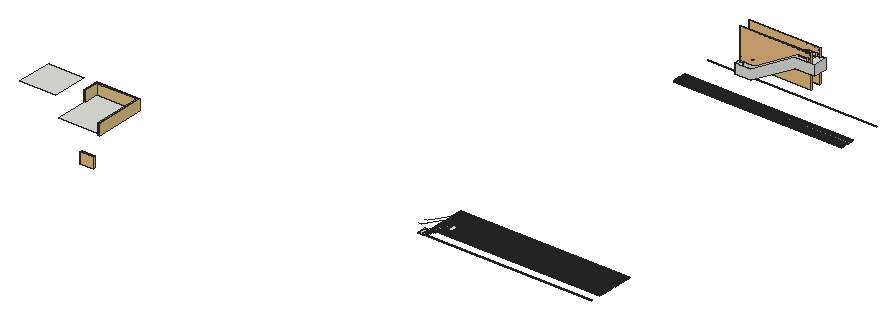
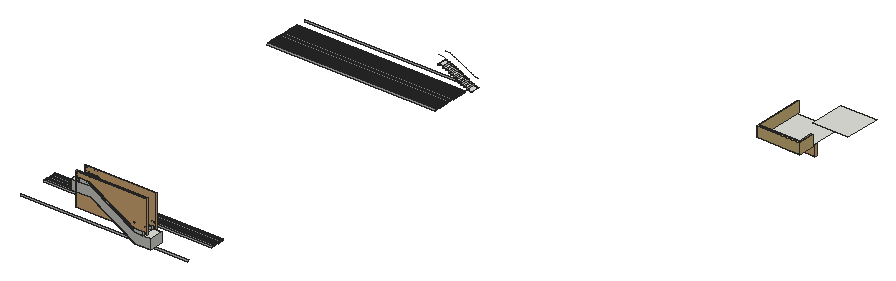
# SketchUp Ruby script. Lengths in inches.
U = 1.inch
M = Sketchup.active_model
def pt(a) = Geom::Point3d.new(a.map { |v| v * U })
def face(e, loops, mat)
  f = e.add_face(loops[0].map { |a| pt(a) })
  loops[1..].each { |l| e.add_face(l.map { |a| pt(a) }).erase! }
  f.material = f.back_material = mat if mat
  f
end
# faces: each face lists its corners as indices into pts; further lists are holes
def faces(e, pts, list, mat = nil) = list.each { |f| face(e, (f[0].is_a?(Array) ? f : [f]).map { |l| l.map { |i| pts[i] } }, mat) }
# xy, xz, yz: faces in a plane at the given z, y or x. An outline is a flat list of corners, or four numbers for a rectangle; further outlines are holes
def ring(l) = l.size == 4 ? [[l[0], l[1]], [l[2], l[1]], [l[2], l[3]], [l[0], l[3]]] : l.each_slice(2).to_a
def flat(e, list, mat, &to3) = list.each { |f| face(e, (f[0].is_a?(Array) ? f : [f]).map { |l| ring(l).map { |u, v| to3.(u, v) } }, mat) }
def xy(e, z, list, mat = nil) = flat(e, list, mat) { |x, y| [x, y, z] }
def xz(e, y, list, mat = nil) = flat(e, list, mat) { |x, z| [x, y, z] }
def yz(e, x, list, mat = nil) = flat(e, list, mat) { |y, z| [x, y, z] }
def lines(e, pts, list) = list.each { |a, b| e.add_line(pt(pts[a]), pt(pts[b])) }
# prism: a flat outline (further loops are holes) pulled along v
def prism(e, loops, v, mat = nil)
  f = face(e, loops, mat); d = Geom::Vector3d.new(v.map { |x| x * U })
  f.pushpull(f.normal.samedirection?(d) ? d.length : -d.length)
end
def box(e, o, s, mat = nil) = prism(e, [[o, [o[0] + s[0], o[1], o[2]], [o[0] + s[0], o[1] + s[1], o[2]], [o[0], o[1] + s[1], o[2]]]], [0, 0, s[2]], mat)
def at(x, y, z, deg = 0) = Geom::Transformation.translation(pt([x, y, z])) * Geom::Transformation.rotation(ORIGIN, Z_AXIS, deg.degrees)
def axes(o, x, y, z) = Geom::Transformation.new([*x, 0, *y, 0, *z, 0, *pt(o).to_a, 1])
def part(name) = M.definitions.add(name)
# library, detail: a bought-in or finely detailed component or shape, given as its bounding box
def library(name, o, s) = part(name).tap { |d| box(d.entities, o, s) }
def detail(e, o, s) = box(e.add_group.entities, o, s)
def put(e, d, t, mat = nil) = e.add_instance(d, t).tap { |i| i.material = mat if mat }
def group(e, t, mat = nil) = e.add_group.tap { |g| g.transformation = t; g.material = mat if mat }.entities
root = M.entities
M.materials.add("[Stone Brushed Khaki]").color = [226, 197, 133]
c1 = part("Group74\#1")
p = [[385.16,-763.86,0],[-385.16,-763.86,0],[-385.16,-767.25,5.875],[385.16,-767.25,5.875]]
faces(c1.entities,p,[[0,1,2,3]])
c2 = part("Group75\#1")
p = [[385.16,-759.92,0],[-385.16,-759.92,0],[-385.16,-763.3125,5.875],[385.16,-763.3125,5.875]]
faces(c2.entities,p,[[0,1,2,3]])
c3 = part("Group76\#1")
p = [[385.16,-755.98,0],[-385.16,-755.98,0],[-385.16,-759.375,5.875],[385.16,-759.375,5.875]]
faces(c3.entities,p,[[0,1,2,3]])
c4 = part("Group77\#1")
p = [[385.16,-752.05,0],[-385.16,-752.05,0],[-385.16,-755.4375,5.875],[385.16,-755.4375,5.875]]
faces(c4.entities,p,[[0,1,2,3]])
c5 = part("Group78\#1")
p = [[385.16,-748.11,0],[-385.16,-748.11,0],[-385.16,-751.5,5.875],[385.16,-751.5,5.875]]
faces(c5.entities,p,[[0,1,2,3]])
c6 = part("Group79\#1")
p = [[385.16,-744.17,0],[-385.16,-744.17,0],[-385.16,-747.5625,5.875],[385.16,-747.5625,5.875]]
faces(c6.entities,p,[[0,1,2,3]])
c7 = part("Group80\#1")
p = [[-385.16,-743.625,5.875],[385.16,-743.625,5.875],[385.16,-740.23,0],[-385.16,-740.23,0]]
faces(c7.entities,p,[[0,1,2,3]])
c8 = part("Group81\#1")
p = [[-385.16,-739.6875,5.875],[385.16,-739.6875,5.875],[385.16,-736.3,0],[-385.16,-736.3,0]]
faces(c8.entities,p,[[0,1,2,3]])
c9 = part("Group82\#1")
p = [[-385.16,-735.75,5.875],[385.16,-735.75,5.875],[385.16,-732.36,0],[-385.16,-732.36,0]]
faces(c9.entities,p,[[0,1,2,3]])
c10 = part("Group83\#1")
p = [[-385.16,-731.8125,5.875],[385.16,-731.8125,5.875],[385.16,-728.42,0],[-385.16,-728.42,0]]
faces(c10.entities,p,[[0,1,2,3]])
c11 = part("Group84\#1")
p = [[385.16,-724.48,0],[-385.16,-724.48,0],[-385.16,-727.875,5.875],[385.16,-727.875,5.875]]
faces(c11.entities,p,[[0,1,2,3]])
c12 = part("Group85\#1")
p = [[385.16,-720.55,0],[-385.16,-720.55,0],[-385.16,-723.9375,5.875],[385.16,-723.9375,5.875]]
faces(c12.entities,p,[[0,1,2,3]])
c13 = part("Group86\#1")
p = [[-385.16,-720,5.875],[385.16,-720,5.875],[385.16,-716.61,0],[-385.16,-716.61,0]]
faces(c13.entities,p,[[0,1,2,3]])
c14 = part("Group88\#1")
p = [[-385.16,-712.125,5.875],[385.16,-712.125,5.875],[385.16,-708.73,0],[-385.16,-708.73,0]]
faces(c14.entities,p,[[0,1,2,3]])
c15 = part("Group90\#1")
p = [[-385.16,-704.25,5.875],[385.16,-704.25,5.875],[385.16,-700.86,0],[-385.16,-700.86,0]]
faces(c15.entities,p,[[0,1,2,3]])
c16 = part("Group92\#1")
p = [[385.16,-692.98,0],[-385.16,-692.98,0],[-385.16,-696.375,5.875],[385.16,-696.375,5.875]]
faces(c16.entities,p,[[0,1,2,3]])
c17 = part("Group94\#1")
p = [[385.16,-685.11,0],[-385.16,-685.11,0],[-385.16,-688.5,5.875],[385.16,-688.5,5.875]]
faces(c17.entities,p,[[0,1,2,3]])
c18 = part("Group96\#1")
p = [[385.16,-677.23,0],[-385.16,-677.23,0],[-385.16,-680.625,5.875],[385.16,-680.625,5.875]]
faces(c18.entities,p,[[0,1,2,3]])
c19 = part("Group98\#1")
p = [[385.16,-669.36,0],[-385.16,-669.36,0],[-385.16,-672.75,5.875],[385.16,-672.75,5.875]]
faces(c19.entities,p,[[0,1,2,3]])
c20 = part("Group100\#1")
p = [[385.16,-661.48,0],[-385.16,-661.48,0],[-385.16,-664.875,5.875],[385.16,-664.875,5.875]]
faces(c20.entities,p,[[0,1,2,3]])
c21 = part("Group101\#1")
p = [[385.16,-657.55,0],[-385.16,-657.55,0],[-385.16,-660.9375,5.875],[385.16,-660.9375,5.875]]
faces(c21.entities,p,[[0,1,2,3]])
c22 = part("Group102\#1")
p = [[385.16,-653.61,0],[-385.16,-653.61,0],[-385.16,-657,5.875],[385.16,-657,5.875]]
faces(c22.entities,p,[[0,1,2,3]])
c23 = part("Group103\#1")
p = [[385.16,-649.67,0],[-385.16,-649.67,0],[-385.16,-653.0625,5.875],[385.16,-653.0625,5.875]]
faces(c23.entities,p,[[0,1,2,3]])
c24 = part("Group104\#1")
p = [[-385.16,-649.125,5.875],[385.16,-649.125,5.875],[385.16,-645.73,0],[-385.16,-645.73,0]]
faces(c24.entities,p,[[0,1,2,3]])
c25 = part("Group105\#1")
p = [[-385.16,-645.1875,5.875],[385.16,-645.1875,5.875],[385.16,-641.8,0],[-385.16,-641.8,0]]
faces(c25.entities,p,[[0,1,2,3]])
c26 = part("Group106\#1")
p = [[385.16,-637.86,0],[-385.16,-637.86,0],[-385.16,-641.25,5.875],[385.16,-641.25,5.875]]
faces(c26.entities,p,[[0,1,2,3]])
c27 = part("Group107\#1")
p = [[-385.16,-637.3125,5.875],[385.16,-637.3125,5.875],[385.16,-633.92,0],[-385.16,-633.92,0]]
faces(c27.entities,p,[[0,1,2,3]])
c28 = part("Group108\#1")
p = [[-385.16,-633.375,5.875],[385.16,-633.375,5.875],[385.16,-629.98,0],[-385.16,-629.98,0]]
faces(c28.entities,p,[[0,1,2,3]])
c29 = part("Group109\#1")
p = [[385.16,-626.05,0],[-385.16,-626.05,0],[-385.16,-629.4375,5.875],[385.16,-629.4375,5.875]]
faces(c29.entities,p,[[0,1,2,3]])
c30 = part("Group110\#1")
p = [[-385.16,-625.5,5.875],[385.16,-625.5,5.875],[385.16,-622.11,0],[-385.16,-622.11,0]]
faces(c30.entities,p,[[0,1,2,3]])
c31 = part("Group111\#1")
p = [[385.16,-618.17,0],[-385.16,-618.17,0],[-385.16,-621.5625,5.875],[385.16,-621.5625,5.875]]
faces(c31.entities,p,[[0,1,2,3]])
c32 = part("Group112\#1")
p = [[-385.16,-617.625,5.875],[385.16,-617.625,5.875],[385.16,-614.23,0],[-385.16,-614.23,0]]
faces(c32.entities,p,[[0,1,2,3]])
c33 = part("Group113\#1")
p = [[385.16,-610.3,0],[-385.16,-610.3,0],[-385.16,-613.6875,5.875],[385.16,-613.6875,5.875]]
faces(c33.entities,p,[[0,1,2,3]])
c34 = part("Group114\#1")
p = [[385.16,-606.36,0],[-385.16,-606.36,0],[-385.16,-609.75,5.875],[385.16,-609.75,5.875]]
faces(c34.entities,p,[[0,1,2,3]])
c35 = part("Group115\#1")
p = [[385.16,-602.42,0],[-385.16,-602.42,0],[-385.16,-605.8125,5.875],[385.16,-605.8125,5.875]]
faces(c35.entities,p,[[0,1,2,3]])
c36 = part("Group116\#1")
p = [[-385.16,-601.875,5.875],[385.16,-601.875,5.875],[385.16,-598.48,0],[-385.16,-598.48,0]]
faces(c36.entities,p,[[0,1,2,3]])
c37 = part("Group117\#1")
p = [[385.16,-594.55,0],[-385.16,-594.55,0],[-385.16,-597.9375,5.875],[385.16,-597.9375,5.875]]
faces(c37.entities,p,[[0,1,2,3]])
c38 = part("Group426\#1")
p = [[-385.16,618.75,5.875],[385.16,618.75,5.875],[385.16,622.14,0],[-385.16,622.14,0]]
faces(c38.entities,p,[[0,1,2,3]])
c39 = part("Group428\#1")
p = [[385.16,630.02,0],[-385.16,630.02,0],[-385.16,626.625,5.875],[385.16,626.625,5.875]]
faces(c39.entities,p,[[0,1,2,3]])
c40 = part("Group430\#1")
p = [[385.16,637.89,0],[-385.16,637.89,0],[-385.16,634.5,5.875],[385.16,634.5,5.875]]
faces(c40.entities,p,[[0,1,2,3]])
c41 = part("Group432\#1")
p = [[385.16,645.77,0],[-385.16,645.77,0],[-385.16,642.375,5.875],[385.16,642.375,5.875]]
faces(c41.entities,p,[[0,1,2,3]])
c42 = part("Group434\#1")
p = [[-385.16,650.25,5.875],[385.16,650.25,5.875],[385.16,653.64,0],[-385.16,653.64,0]]
faces(c42.entities,p,[[0,1,2,3]])
c43 = part("Group436\#1")
p = [[-385.16,658.125,5.875],[385.16,658.125,5.875],[385.16,661.52,0],[-385.16,661.52,0]]
faces(c43.entities,p,[[0,1,2,3]])
c44 = part("Group438\#1")
p = [[385.16,669.39,0],[-385.16,669.39,0],[-385.16,666,5.875],[385.16,666,5.875]]
faces(c44.entities,p,[[0,1,2,3]])
c45 = part("Group440\#1")
p = [[385.16,677.27,0],[-385.16,677.27,0],[-385.16,673.875,5.875],[385.16,673.875,5.875]]
faces(c45.entities,p,[[0,1,2,3]])
c46 = part("Group442\#1")
p = [[385.16,685.14,0],[-385.16,685.14,0],[-385.16,681.75,5.875],[385.16,681.75,5.875]]
faces(c46.entities,p,[[0,1,2,3]])
c47 = part("Group62\#1")
p = [[385.16,-811.11,0],[-385.16,-811.11,0],[-385.16,-814.5,5.875],[385.16,-814.5,5.875]]
faces(c47.entities,p,[[0,1,2,3]])
c48 = part("Group87\#1")
p = [[385.16,-712.67,0],[-385.16,-712.67,0],[-385.16,-716.0625,5.875],[385.16,-716.0625,5.875]]
faces(c48.entities,p,[[0,1,2,3]])
c49 = part("Group89\#1")
p = [[-385.16,-708.1875,5.875],[385.16,-708.1875,5.875],[385.16,-704.8,0],[-385.16,-704.8,0]]
faces(c49.entities,p,[[0,1,2,3]])
c50 = part("Group476\#1")
p = [[-385.16,815.625,5.875],[385.16,815.625,5.875],[385.16,818.4375,1],[-385.16,818.4375,1]]
faces(c50.entities,p,[[0,1,2,3]])
c51 = part("Group47\#1")
p = [[1638.72,475.15,257.625],[1638.72,451.52,257.625],[1638.72,333.4,198.875],[1638.72,321.59,198.875],[1674.22,475.15,257.625],[1674.22,451.52,257.625],
  [1674.22,333.4,198.875],[1674.22,321.59,198.875]]
lines(c51.entities,p,[[0,1],[1,2],[2,3],[4,5],[5,6],[6,7]])
c52 = part("Group46\#1")
prism(c52.entities,[[[1636.78,475.15,219.25],[1636.78,475.15,218.25],[1636.78,452.52,218.25],[1636.78,452.52,212.375],[1636.78,440.71,212.375],[1636.78,440.71,206.5],[1636.78,428.9,206.5],[1636.78,428.9,200.625],[1636.78,417.09,200.625],[1636.78,417.09,194.75],[1636.78,405.27,194.75],[1636.78,405.27,188.875],[1636.78,393.46,188.875],[1636.78,393.46,183],[1636.78,381.65,183],[1636.78,381.65,177.125],[1636.78,369.84,177.125],[1636.78,369.84,171.25],[1636.78,358.02,171.25],[1636.78,358.02,165.375],[1636.78,346.21,165.375],[1636.78,346.21,159.5],[1636.78,321.59,159.5],[1636.78,321.59,160.5],[1636.78,345.21,160.5],[1636.78,345.21,166.375],[1636.78,357.02,166.375],[1636.78,357.02,172.25],[1636.78,368.84,172.25],[1636.78,368.84,178.125],[1636.78,380.65,178.125],[1636.78,380.65,184],[1636.78,392.46,184],[1636.78,392.46,189.875],[1636.78,404.27,189.875],[1636.78,404.27,195.75],[1636.78,416.09,195.75],[1636.78,416.09,201.625],[1636.78,427.9,201.625],[1636.78,427.9,207.5],[1636.78,439.71,207.5],[1636.78,439.71,213.375],[1636.78,451.52,213.375],[1636.78,451.52,219.25]]],[39.375,0,0])
put(c52.entities,c51,at(0,0,0))
c53 = library("Group\#7",[0,0,0],[62.33,9.07,48])
c54 = part("Group49\#1")
xy(c54.entities,-45.98,[[-72.01,-31.5,0,31.5]])
xy(c54.entities,72.125,[[204.57,-31.5,294.57,31.5]])
xz(c54.entities,-31.5,[[-72.01,-45.98,0,-45.98,204.57,72.125,294.57,72.125,294.57,118.11,204.57,118.11,0,0,-72.01,0]])
xz(c54.entities,31.5,[[-72.01,-45.98,-72.01,0,0,0,204.57,118.11,294.57,118.11,294.57,72.125,204.57,72.125,0,-45.98]])
yz(c54.entities,-72.01,[[-31.5,-45.98,31.5,0]])
yz(c54.entities,294.57,[[-31.5,72.125,31.5,118.11]])
p = [[0,-31.5,-45.98],[0,31.5,-45.98],[204.57,31.5,72.125],[204.57,-31.5,72.125]]
faces(c54.entities,p,[[0,1,2,3]])
c55 = part("Group50\#1")
prism(c55.entities,[[[-35.98,-31.5,14.02],[-35.98,-31.5,0],[0,-31.5,0],[204.57,-31.5,118.11],[258.59,-31.5,118.11],[258.59,-31.5,132.125],[223.27,-31.5,132.125],[222.02,-31.5,132.09],[220.76,-31.5,131.99],[219.52,-31.5,131.83],[218.28,-31.5,131.6],[217.06,-31.5,131.31],[215.85,-31.5,130.95],[214.67,-31.5,130.53],[213.51,-31.5,130.05],[212.37,-31.5,129.51],[211.27,-31.5,128.91],[23.41,-31.5,20.45],[21.2,-31.5,19.25],[18.93,-31.5,18.16],[16.61,-31.5,17.2],[14.24,-31.5,16.36],[11.83,-31.5,15.65],[9.39,-31.5,15.0625],[6.92,-31.5,14.61],[4.43,-31.5,14.28],[1.92,-31.5,14.08],[-0.59,-31.5,14.02]]],[0,11.8125,0])
c56 = part("Group51\#1")
prism(c56.entities,[[[-38.42,-26,8.24],[-37.21,-26,8.08],[-35.98,-26,8.03],[-35.98,-26,14.02],[-0.59,-26,14.02],[3.6,-26,14.2],[7.75,-26,14.75],[11.84,-26,15.65],[15.84,-26,16.91],[19.71,-26,18.52],[23.43,-26,20.45],[211.27,-26,128.91],[213.125,-26,129.875],[215.06,-26,130.68],[217.06,-26,131.31],[219.1,-26,131.76],[221.18,-26,132.03],[223.27,-26,132.125],[258.59,-26,132.125],[258.59,-26,126.14],[259.81,-26,126.2],[261.02,-26,126.35],[262.22,-26,126.62],[263.38,-26,126.99],[264.51,-26,127.45],[265.6,-26,128.02],[266.63,-26,128.68],[267.6,-26,129.42],[268.5,-26,130.25],[269.33,-26,131.15],[270.07,-26,132.12],[270.73,-26,133.15],[271.29,-26,134.23],[271.76,-26,135.36],[272.125,-26,136.53],[272.39,-26,137.72],[272.55,-26,138.9375],[272.6,-26,140.16],[272.55,-26,141.38],[272.39,-26,142.59],[272.125,-26,143.79],[271.76,-26,144.95],[271.29,-26,146.08],[270.73,-26,147.17],[270.07,-26,148.2],[269.33,-26,149.17],[268.5,-26,150.07],[267.6,-26,150.89],[266.63,-26,151.64],[265.6,-26,152.3],[264.51,-26,152.86],[263.38,-26,153.33],[262.22,-26,153.7],[261.02,-26,153.96],[259.81,-26,154.12],[258.59,-26,154.17],[223.27,-26,154.17],[219.26,-26,154],[215.27,-26,153.47],[211.35,-26,152.6],[207.52,-26,151.4],[203.81,-26,149.86],[200.24,-26,148],[12.4,-26,39.54],[10.39,-26,38.5],[8.3,-26,37.63],[6.13,-26,36.95],[3.92,-26,36.46],[1.67,-26,36.16],[-0.59,-26,36.0625],[-35.98,-26,36.0625],[-37.21,-26,36.01],[-38.42,-26,35.85],[-39.61,-26,35.59],[-40.78,-26,35.22],[-41.91,-26,34.75],[-42.99,-26,34.19],[-44.02,-26,33.53],[-44.99,-26,32.78],[-45.89,-26,31.96],[-46.72,-26,31.06],[-47.47,-26,30.09],[-48.12,-26,29.06],[-48.6875,-26,27.97],[-49.15,-26,26.84],[-49.52,-26,25.67],[-49.79,-26,24.48],[-49.95,-26,23.27],[-50,-26,22.05],[-49.95,-26,20.83],[-49.79,-26,19.61],[-49.52,-26,18.42],[-49.15,-26,17.25],[-48.6875,-26,16.125],[-48.12,-26,15.04],[-47.47,-26,14.01],[-46.72,-26,13.04],[-45.89,-26,12.14],[-44.99,-26,11.3125],[-44.02,-26,10.57],[-42.99,-26,9.91],[-41.91,-26,9.34],[-40.78,-26,8.875],[-39.61,-26,8.51]]],[0,0.8125,0])
c57 = library("Group52\#1",[-51.57,-27.17,6.46],[325.75,3.15,149.29])
c58 = part("Group53\#1")
xy(c58.entities,0,[[-35.98,-19.6875,-24.93,19.6875],[-24.93,-19.6875,-8.07,19.6875],[-8.07,-19.6875,8.8,19.6875]])
xy(c58.entities,4.72,[[8.18,-19.6875,25.05,19.6875]])
xy(c58.entities,13.78,[[23.87,-19.6875,40.73,19.6875]])
xy(c58.entities,22.83,[[39.55,-19.6875,56.42,19.6875]])
xy(c58.entities,31.89,[[55.23,-19.6875,72.1,19.6875]])
xy(c58.entities,40.94,[[70.92,-19.6875,87.78,19.6875]])
xy(c58.entities,50,[[86.6,-19.6875,103.47,19.6875]])
xy(c58.entities,59.06,[[102.29,-19.6875,119.15,19.6875]])
xy(c58.entities,68.11,[[117.97,-19.6875,134.84,19.6875]])
xy(c58.entities,77.17,[[133.65,-19.6875,150.52,19.6875]])
xy(c58.entities,86.22,[[149.34,-19.6875,166.2,19.6875]])
xy(c58.entities,95.28,[[165.02,-19.6875,181.89,19.6875]])
xy(c58.entities,104.33,[[180.71,-19.6875,197.57,19.6875]])
xy(c58.entities,113.39,[[196.39,-19.6875,213.26,19.6875]])
xy(c58.entities,118.11,[[212.64,-19.6875,229.5,19.6875],[229.5,-19.6875,246.37,19.6875],[246.37,-19.6875,258.59,19.6875]])
p = [[8.18,-19.6875,4.72],[8.18,19.6875,4.72],[8.8,19.6875,0],[8.8,-19.6875,0],[23.87,-19.6875,13.78],[23.87,19.6875,13.78],
  [25.05,19.6875,4.72],[25.05,-19.6875,4.72],[39.55,-19.6875,22.83],[39.55,19.6875,22.83],[40.73,19.6875,13.78],[40.73,-19.6875,13.78],
  [55.23,-19.6875,31.89],[55.23,19.6875,31.89],[56.42,19.6875,22.83],[56.42,-19.6875,22.83],[70.92,-19.6875,40.94],[70.92,19.6875,40.94],
  [72.1,19.6875,31.89],[72.1,-19.6875,31.89],[86.6,-19.6875,50],[86.6,19.6875,50],[87.78,19.6875,40.94],[87.78,-19.6875,40.94],
  [102.29,-19.6875,59.06],[102.29,19.6875,59.06],[103.47,19.6875,50],[103.47,-19.6875,50],[117.97,-19.6875,68.11],[117.97,19.6875,68.11],
  [119.15,19.6875,59.06],[119.15,-19.6875,59.06],[133.65,-19.6875,77.17],[133.65,19.6875,77.17],[134.84,19.6875,68.11],[134.84,-19.6875,68.11],
  [149.34,-19.6875,86.22],[149.34,19.6875,86.22],[150.52,19.6875,77.17],[150.52,-19.6875,77.17],[165.02,-19.6875,95.28],[165.02,19.6875,95.28],
  [166.2,19.6875,86.22],[166.2,-19.6875,86.22],[180.71,-19.6875,104.33],[180.71,19.6875,104.33],[181.89,19.6875,95.28],[181.89,-19.6875,95.28],
  [196.39,-19.6875,113.39],[196.39,19.6875,113.39],[197.57,19.6875,104.33],[197.57,-19.6875,104.33],[212.64,-19.6875,118.11],[212.64,19.6875,118.11],
  [213.26,19.6875,113.39],[213.26,-19.6875,113.39]]
faces(c58.entities,p,[[0,1,2,3],[4,5,6,7],[8,9,10,11],[12,13,14,15],[16,17,18,19],[20,21,22,23],[24,25,26,27],[28,29,30,31],
  [32,33,34,35],[36,37,38,39],[40,41,42,43],[44,45,46,47],[48,49,50,51],[52,53,54,55]])
c59 = part("Group54\#1")
xz(c59.entities,-19.6875,[[-35.98,-19.69,-35.98,0,0,0,204.57,118.11,258.59,118.11,258.59,98.43,204.57,98.43,0,-19.69]])
xz(c59.entities,19.6875,[[-35.98,-19.69,0,-19.69,204.57,98.43,258.59,98.43,258.59,118.11,204.57,118.11,0,0,-35.98,0]])
p = [[0,-19.6875,0],[0,-31.5,0],[204.57,-31.5,118.11],[204.57,-19.6875,118.11],[0,19.6875,0],[0,31.5,0],
  [204.57,31.5,118.11],[204.57,19.6875,118.11]]
faces(c59.entities,p,[[0,1,2,3],[4,5,6,7]])
c60 = part("Group55\#1")
xy(c60.entities,0,[[-72.01,-31.5,0,-31.5,0,-19.6875,-35.98,-19.6875,-35.98,19.6875,0,19.6875,0,31.5,-72.01,31.5]])
xy(c60.entities,118.11,[[204.57,-31.5,294.57,-31.5,294.57,31.5,204.57,31.5,204.57,19.6875,258.59,19.6875,258.59,-19.6875,204.57,-19.6875]])
c61 = part("Group50\#2")
prism(c61.entities,[[[-35.98,-31.5,14.02],[-35.98,-31.5,0],[0,-31.5,0],[204.57,-31.5,118.11],[258.59,-31.5,118.11],[258.59,-31.5,132.125],[223.27,-31.5,132.125],[222.02,-31.5,132.09],[220.76,-31.5,131.99],[219.52,-31.5,131.83],[218.28,-31.5,131.6],[217.06,-31.5,131.31],[215.85,-31.5,130.95],[214.67,-31.5,130.53],[213.51,-31.5,130.05],[212.37,-31.5,129.51],[211.27,-31.5,128.91],[23.41,-31.5,20.45],[21.2,-31.5,19.25],[18.93,-31.5,18.16],[16.61,-31.5,17.2],[14.24,-31.5,16.36],[11.83,-31.5,15.65],[9.39,-31.5,15.0625],[6.92,-31.5,14.61],[4.43,-31.5,14.28],[1.92,-31.5,14.08],[-0.59,-31.5,14.02]]],[0,11.8125,0])
c62 = part("Group51\#2")
prism(c62.entities,[[[-38.42,-26,8.24],[-37.21,-26,8.08],[-35.98,-26,8.03],[-35.98,-26,14.02],[-0.59,-26,14.02],[3.6,-26,14.2],[7.75,-26,14.75],[11.84,-26,15.65],[15.84,-26,16.91],[19.71,-26,18.52],[23.43,-26,20.45],[211.27,-26,128.91],[213.125,-26,129.875],[215.06,-26,130.68],[217.06,-26,131.31],[219.1,-26,131.76],[221.18,-26,132.03],[223.27,-26,132.125],[258.59,-26,132.125],[258.59,-26,126.14],[259.81,-26,126.2],[261.02,-26,126.35],[262.22,-26,126.62],[263.38,-26,126.99],[264.51,-26,127.45],[265.6,-26,128.02],[266.63,-26,128.68],[267.6,-26,129.42],[268.5,-26,130.25],[269.33,-26,131.15],[270.07,-26,132.12],[270.73,-26,133.15],[271.29,-26,134.23],[271.76,-26,135.36],[272.125,-26,136.53],[272.39,-26,137.72],[272.55,-26,138.9375],[272.6,-26,140.16],[272.55,-26,141.38],[272.39,-26,142.59],[272.125,-26,143.79],[271.76,-26,144.95],[271.29,-26,146.08],[270.73,-26,147.17],[270.07,-26,148.2],[269.33,-26,149.17],[268.5,-26,150.07],[267.6,-26,150.89],[266.63,-26,151.64],[265.6,-26,152.3],[264.51,-26,152.86],[263.38,-26,153.33],[262.22,-26,153.7],[261.02,-26,153.96],[259.81,-26,154.12],[258.59,-26,154.17],[223.27,-26,154.17],[219.26,-26,154],[215.27,-26,153.47],[211.35,-26,152.6],[207.52,-26,151.4],[203.81,-26,149.86],[200.24,-26,148],[12.4,-26,39.54],[10.39,-26,38.5],[8.3,-26,37.63],[6.13,-26,36.95],[3.92,-26,36.46],[1.67,-26,36.16],[-0.59,-26,36.0625],[-35.98,-26,36.0625],[-37.21,-26,36.01],[-38.42,-26,35.85],[-39.61,-26,35.59],[-40.78,-26,35.22],[-41.91,-26,34.75],[-42.99,-26,34.19],[-44.02,-26,33.53],[-44.99,-26,32.78],[-45.89,-26,31.96],[-46.72,-26,31.06],[-47.47,-26,30.09],[-48.12,-26,29.06],[-48.6875,-26,27.97],[-49.15,-26,26.84],[-49.52,-26,25.67],[-49.79,-26,24.48],[-49.95,-26,23.27],[-50,-26,22.05],[-49.95,-26,20.83],[-49.79,-26,19.61],[-49.52,-26,18.42],[-49.15,-26,17.25],[-48.6875,-26,16.125],[-48.12,-26,15.04],[-47.47,-26,14.01],[-46.72,-26,13.04],[-45.89,-26,12.14],[-44.99,-26,11.3125],[-44.02,-26,10.57],[-42.99,-26,9.91],[-41.91,-26,9.34],[-40.78,-26,8.875],[-39.61,-26,8.51]]],[0,0.8125,0])
c63 = library("Group52\#2",[-51.57,-27.17,6.46],[325.75,3.15,149.29])
c64 = part("Group48\#1")
put(c64.entities,c54,at(0,0,0))
put(c64.entities,c55,at(0,0,0))
put(c64.entities,c56,at(0,0,0))
put(c64.entities,c57,at(0,0,0))
put(c64.entities,c58,at(0,0,0))
put(c64.entities,c59,at(0,0,0))
put(c64.entities,c60,at(0,0,0))
put(c64.entities,c61,at(0,51.1875,0))
put(c64.entities,c62,at(0,51.1875,0))
put(c64.entities,c63,at(0,51.1875,0))
xy(root,308.1875,[[171,57.4375,354,273.4375]])
xy(root,308.1875,[[354,48.4375,354,273.4375,171,273.4375,171,210.3,162,210.3,162,282.4375,363,282.4375,363,48.4375]],"[Stone Brushed Khaki]")
xy(root,356.1875,[[354,48.4375,363,48.4375,363,282.4375,162,282.4375,162,210.3,171,210.3,171,273.4375,354,273.4375]],"[Stone Brushed Khaki]")
xy(root,405.6875,[[0,48.4375,162,210.4375]])
xz(root,48.4375,[[354,308.1875,363,356.1875]],"[Stone Brushed Khaki]")
xz(root,210.3,[[162,308.1875,171,356.1875]],"[Stone Brushed Khaki]")
xz(root,273.4375,[[171,308.1875,354,356.1875]],"[Stone Brushed Khaki]")
xz(root,282.4375,[[162,308.1875,363,356.1875]],"[Stone Brushed Khaki]")
yz(root,162,[[210.3,308.1875,282.4375,356.1875]],"[Stone Brushed Khaki]")
yz(root,171,[[210.3,308.1875,273.4375,356.1875]],"[Stone Brushed Khaki]")
yz(root,354,[[48.4375,308.1875,273.4375,356.1875]],"[Stone Brushed Khaki]")
yz(root,363,[[48.4375,308.1875,282.4375,356.1875]],"[Stone Brushed Khaki]")
put(root,c1,at(1937.93,1232.46,154.625))
put(root,c2,at(1937.93,1232.46,154.625))
put(root,c3,at(1937.93,1232.46,154.625))
put(root,c4,at(1937.93,1232.46,154.625))
put(root,c5,at(1937.93,1232.46,154.625))
put(root,c6,at(1937.93,1232.46,154.625))
put(root,c7,at(1937.93,1232.46,154.625))
put(root,c8,at(1937.93,1232.46,154.625))
put(root,c9,at(1937.93,1232.46,154.625))
put(root,c10,at(1937.93,1232.46,154.625))
put(root,c11,at(1937.93,1232.46,154.625))
put(root,c12,at(1937.93,1232.46,154.625))
put(root,c13,at(1937.93,1232.46,154.625))
put(root,c14,at(1937.93,1232.46,154.625))
put(root,c15,at(1937.93,1232.46,154.625))
put(root,c16,at(1937.93,1232.46,154.625))
put(root,c17,at(1937.93,1232.46,154.625))
put(root,c18,at(1937.93,1232.46,154.625))
put(root,c19,at(1937.93,1232.46,154.625))
put(root,c20,at(1937.93,1232.46,154.625))
put(root,c21,at(1937.93,1232.46,154.625))
put(root,c22,at(1937.93,1232.46,154.625))
put(root,c23,at(1937.93,1232.46,154.625))
put(root,c24,at(1937.93,1232.46,154.625))
put(root,c25,at(1937.93,1232.46,154.625))
put(root,c26,at(1937.93,1232.46,154.625))
put(root,c27,at(1937.93,1232.46,154.625))
put(root,c28,at(1937.93,1232.46,154.625))
put(root,c29,at(1937.93,1232.46,154.625))
put(root,c30,at(1937.93,1232.46,154.625))
put(root,c31,at(1937.93,1232.46,154.625))
put(root,c32,at(1937.93,1232.46,154.625))
put(root,c33,at(1937.93,1232.46,154.625))
put(root,c34,at(1937.93,1232.46,154.625))
put(root,c35,at(1937.93,1232.46,154.625))
put(root,c36,at(1937.93,1232.46,154.625))
put(root,c37,at(1937.93,1232.46,154.625))
put(root,c38,at(1937.93,1232.46,154.625))
put(root,c39,at(1937.93,1232.46,154.625))
put(root,c40,at(1937.93,1232.46,154.625))
put(root,c41,at(1937.93,1232.46,154.625))
put(root,c42,at(1937.93,1232.46,154.625))
put(root,c43,at(1937.93,1232.46,154.625))
put(root,c44,at(1937.93,1232.46,154.625))
put(root,c45,at(1937.93,1232.46,154.625))
put(root,c46,at(1937.93,1232.46,154.625))
put(root,c47,at(1937.93,1232.46,154.625))
put(root,c48,at(1937.93,1232.46,154.625))
put(root,c49,at(1937.93,1232.46,154.625))
put(root,c50,at(1937.93,1232.46,154.625))
put(root,c52,at(1209.38,2090.18,0,-90))
put(root,c53,at(273.34,48.4375,162))
put(root,c64,at(1771.15,2050.9,213.16))
